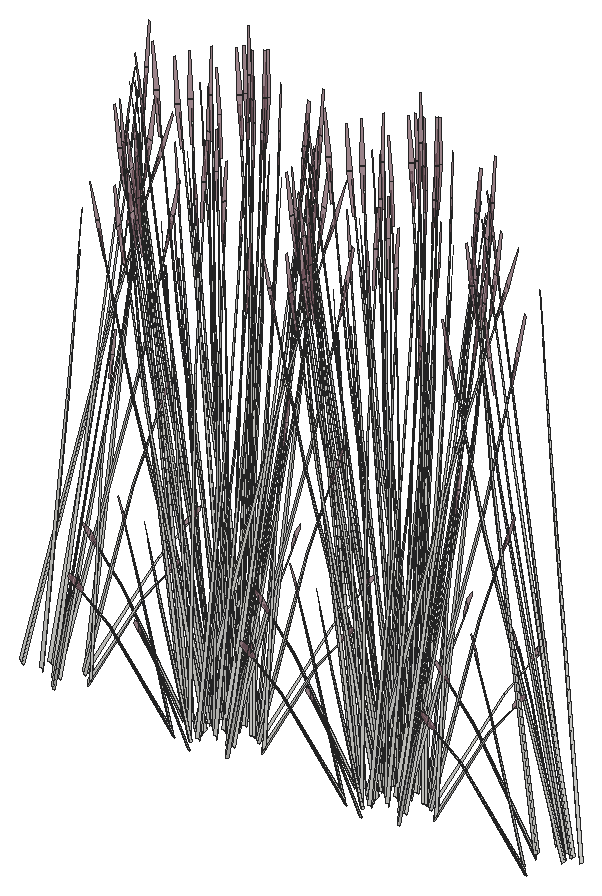
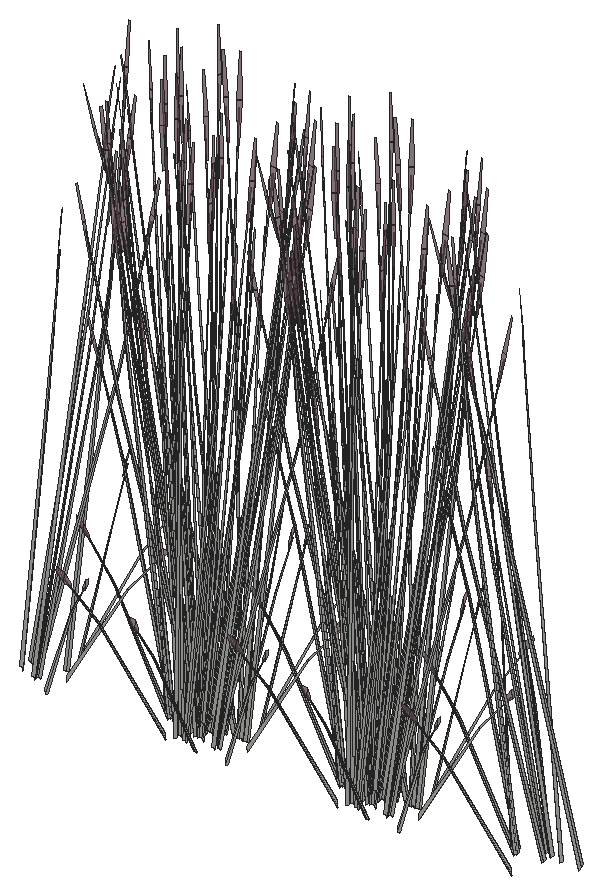
# SketchUp Ruby script. Lengths in inches.
U = 1.inch
M = Sketchup.active_model
def pt(a) = Geom::Point3d.new(a.map { |v| v * U })
def face(e, loops, mat)
  f = e.add_face(loops[0].map { |a| pt(a) })
  loops[1..].each { |l| e.add_face(l.map { |a| pt(a) }).erase! }
  f.material = f.back_material = mat if mat
  f
end
# faces: each face lists its corners as indices into pts; further lists are holes
def faces(e, pts, list, mat = nil) = list.each { |f| face(e, (f[0].is_a?(Array) ? f : [f]).map { |l| l.map { |i| pts[i] } }, mat) }
# xy, xz, yz: faces in a plane at the given z, y or x. An outline is a flat list of corners, or four numbers for a rectangle; further outlines are holes
def ring(l) = l.size == 4 ? [[l[0], l[1]], [l[2], l[1]], [l[2], l[3]], [l[0], l[3]]] : l.each_slice(2).to_a
def flat(e, list, mat, &to3) = list.each { |f| face(e, (f[0].is_a?(Array) ? f : [f]).map { |l| ring(l).map { |u, v| to3.(u, v) } }, mat) }
def xy(e, z, list, mat = nil) = flat(e, list, mat) { |x, y| [x, y, z] }
def xz(e, y, list, mat = nil) = flat(e, list, mat) { |x, z| [x, y, z] }
def yz(e, x, list, mat = nil) = flat(e, list, mat) { |y, z| [x, y, z] }
def lines(e, pts, list) = list.each { |a, b| e.add_line(pt(pts[a]), pt(pts[b])) }
# prism: a flat outline (further loops are holes) pulled along v
def prism(e, loops, v, mat = nil)
  f = face(e, loops, mat); d = Geom::Vector3d.new(v.map { |x| x * U })
  f.pushpull(f.normal.samedirection?(d) ? d.length : -d.length)
end
def box(e, o, s, mat = nil) = prism(e, [[o, [o[0] + s[0], o[1], o[2]], [o[0] + s[0], o[1] + s[1], o[2]], [o[0], o[1] + s[1], o[2]]]], [0, 0, s[2]], mat)
def at(x, y, z, deg = 0) = Geom::Transformation.translation(pt([x, y, z])) * Geom::Transformation.rotation(ORIGIN, Z_AXIS, deg.degrees)
def axes(o, x, y, z) = Geom::Transformation.new([*x, 0, *y, 0, *z, 0, *pt(o).to_a, 1])
def part(name) = M.definitions.add(name)
# library, detail: a bought-in or finely detailed component or shape, given as its bounding box
def library(name, o, s) = part(name).tap { |d| box(d.entities, o, s) }
def detail(e, o, s) = box(e.add_group.entities, o, s)
def put(e, d, t, mat = nil) = e.add_instance(d, t).tap { |i| i.material = mat if mat }
def group(e, t, mat = nil) = e.add_group.tap { |g| g.transformation = t; g.material = mat if mat }.entities
root = M.entities
M.materials.add("LightPink_Translucent").color = [144, 107, 117]
M.materials["LightPink_Translucent"].alpha = 0.75
c1 = part("blade")
p = [[2.15,0.21,22],[0,0.17,0],[0.09,0.45,0],[2.18,0.31,22],[2.29,0.31,22],[0.38,0.45,0],
  [2.48,0.24,33],[2.49,0.24,33],[2.48,0.22,33]]
faces(c1.entities,p,[[0,1,2,3],[4,5,2,3],[6,3,4,7],[8,0,3,6]])
c2 = part("seeds")
p = [[0.3,-0.1,1.38],[-0.01,-0.03,1.59],[-0.01,-0.03,0.03],[0.14,-0.07,-0.07],[0.29,-0.03,3],[0.15,0.01,3.11]]
faces(c2.entities,p,[[0,1,2,3],[1,0,4,5]],"LightPink_Translucent")
c3 = part("blade with seeds")
put(c3.entities,c1,at(0,0,0))
put(c3.entities,c2,axes([2.4,0.25,30.99],[1.5799,-0.05474,1.17369],[-0.12525,1.92788,0.29478],[-0.07173,-0.02425,1.56792]))
put(root,c3,axes([309.91,52.51,257.06],[0.51177,-0.45928,-0.62353],[0.63575,0.41646,-0.16365],[0.20507,-0.11457,1.37633]))
put(root,c3,axes([312.16,52.1,257.03],[0.17848,0.53243,-0.30978],[-0.70886,0.15119,0.30978],[0.1429,0.0614,1.38974]))
put(root,c3,axes([313.49,53.84,257.375],[0.95008,0,0],[0,0.68292,-0.51607],[0,0.15554,1.63711]))
put(root,c3,axes([310.42,52.95,257.67],[0.76714,-0.40567,-0.29095],[0.51013,0.57321,-0.50002],[0.18927,0.05821,1.59708]))
put(root,c3,axes([308.49,52.59,256.59],[-0.74787,0.24464,1.28929],[-0.23804,-0.70192,0.50096],[0.45924,0.01168,1.46642]))
put(root,c3,axes([311.92,51.51,257.375],[0.47504,-0.61229,0],[0.79476,0.34146,-0.51607],[0.18101,0.07777,1.63711]))
put(root,c3,axes([312.72,51.24,256.49],[-0.11372,-0.04814,1.76342],[-0.29211,-0.53779,-0.26939],[0.19706,-0.14594,0.30037]))
put(root,c3,axes([312.36,51.875,257.02],[0.7111,0.30552,-0.49651],[-0.42504,0.54784,0],[0.16196,0.06958,1.57504]))
put(root,c3,axes([312.32,56.22,256.49],[0.05536,-0.08822,1.76342],[0.69692,-0.25981,-0.26939],[0.21129,0.13447,0.30037]))
put(root,c3,axes([311.32,53.05,257.06],[0.79037,0.10018,-0.62353],[-0.16679,0.61794,-0.16365],[0.23587,0.07488,1.37633]))
put(root,c3,axes([314.6875,53.41,257.26],[-0.47106,-0.39072,-0.06488],[0.51591,-0.35801,-0.29416],[0.14618,-0.02521,0.97024]))
put(root,c3,axes([324.24,53.45,256.49],[0.01927,0.0963,1.76342],[-0.38846,0.5029,-0.26939],[-0.27592,-0.02535,0.30037]))
put(root,c3,axes([313.79,53.93,256.98],[-0.48937,0.07333,1.41583],[-0.07789,-0.58369,0.08104],[0.34275,-0.08835,0.80566]))
put(root,c3,axes([314.33,53.55,256.49],[-0.03971,-0.09277,1.76342],[0.27541,-0.54264,-0.26939],[0.27782,-0.00781,0.30037]))
put(root,c3,axes([324.03,56.15,256.49],[0.10192,0.06105,1.76342],[0.17281,0.56562,-0.26939],[-0.22588,0.12062,0.30037]))
put(root,c3,axes([326.78,54.32,257.06],[-0.79037,-0.10018,-0.62353],[0.16679,-0.61794,-0.16365],[-0.23587,-0.07488,1.37633]))
put(root,c3,axes([325.74,55.49,257.02],[-0.7111,-0.30552,-0.49651],[0.42504,-0.54784,0],[-0.16196,-0.06958,1.57504]))
put(root,c3,axes([325.43,50.94,256.49],[-0.0736,0.08049,1.76342],[-0.74378,0.17355,-0.26939],[-0.17968,-0.15788,0.30037]))
put(root,c3,axes([326.17,55.86,257.375],[-0.47504,0.61229,0],[-0.79476,-0.34146,-0.51607],[-0.18101,-0.07777,1.63711]))
put(root,c3,axes([324.97,51.25,257.13],[-0.21918,0.49894,-0.03893],[-0.6746,-0.15348,-0.17649],[-0.10242,-0.08161,0.58215]))
put(root,c3,axes([327.67,54.42,257.67],[-0.76714,0.40567,-0.29095],[-0.51013,-0.57321,-0.50002],[-0.18927,-0.05821,1.59708]))
put(root,c3,axes([324.6,53.53,257.375],[-0.95008,0,0],[0,-0.68292,-0.51607],[0,-0.15554,1.63711]))
put(root,c3,axes([325.9375,55.27,257.03],[-0.17848,-0.53243,-0.30978],[0.70886,-0.15119,0.30978],[-0.1429,-0.0614,1.38974]))
put(root,c3,axes([328.18,54.86,257.06],[-0.51177,0.45928,-0.62353],[-0.63575,-0.41646,-0.16365],[-0.20507,0.11457,1.37633]))
put(root,c3,axes([325.34,53.35,257.33],[-0.70674,0.51372,0.30756],[-0.70717,-0.50832,-0.36492],[-0.02468,-0.14589,1.64885]))
put(root,c3,axes([328.54,54.6,257.46],[-0.74193,-0.49181,-0.25192],[0.6243,-0.55226,0.5513],[-0.19979,0.05753,1.68216]))
put(root,c3,axes([327.1875,54.13,257.21],[-0.45644,-0.51287,-0.44739],[0.69137,-0.36116,0.21531],[-0.14771,-0.06346,1.43643]))
put(root,c3,axes([328.16,54.5,257.21],[-0.82508,0.03772,-0.44739],[-0.07462,-0.62614,0.21531],[-0.14771,0.06346,1.43643]))
put(root,c3,axes([327.25,54.42,257.4375],[0.20138,-0.72405,-0.23429],[0.95485,0.12621,0.51271],[-0.16685,-0.09999,1.5644]))
put(root,c3,axes([329.03,56.11,257.02],[-0.7111,0.30552,-0.49651],[-0.42504,-0.54784,0],[-0.16196,0.06958,1.57504]))
put(root,c3,axes([324.82,53.07,257.02],[0,-0.61104,-0.49651],[0.85008,0,0],[0,-0.13917,1.57504]))
put(root,c3,axes([329.07,55.95,257.19],[-0.46912,-0.61443,-0.05142],[0.79476,-0.34146,0.51607],[-0.19584,0.0585,1.6363]))
put(root,c3,axes([328.86,55.87,257.03],[-0.70886,-0.15119,-0.30978],[0.17848,-0.53243,0.30978],[-0.1429,0.0614,1.38974]))
put(root,c3,axes([327.04,53.77,257.67],[-0.85568,-0.29155,-0.29095],[0.41201,-0.61537,-0.50002],[-0.02689,-0.15109,1.59708]))
put(root,c3,axes([328.74,54.33,257.67],[0.08854,0.69723,-0.29095],[-0.92215,0.04216,-0.50002],[-0.16238,0.09287,1.59708]))
put(root,c3,axes([326.66,53.15,257.1],[-0.31203,-0.62659,-0.69835],[0.89884,-0.22566,-0.18329],[-0.03449,-0.21218,1.54149]))
put(root,c3,axes([325.18,53.08,257.03],[0.53038,-0.38124,-0.30978],[0.53038,0.38124,0.30978],[0,-0.1228,1.38974]))
put(root,c3,axes([327.58,50.62,257.13],[-0.52505,0.35054,-0.03893],[-0.48109,-0.38392,-0.17649],[-0.03387,-0.10878,0.58215]))
put(root,c3,axes([327.9,55.33,257.2],[-0.76598,-0.27433,0],[0.36864,-0.57001,0],[0,0,1.62707]))
put(root,c3,axes([329.67,56.02,257.375],[0.47504,0.61229,0],[-0.79476,0.34146,-0.51607],[-0.18101,0.07777,1.63711]))
put(root,c3,axes([328.71,54.01,257.3],[-0.70674,-0.52593,-0.06131],[0.70717,-0.52625,0],[-0.02468,-0.01837,1.75571]))
put(root,c3,axes([329.1,55.63,257.33],[0.95122,0.19861,0.30756],[-0.23797,0.7099,-0.36492],[-0.15744,0.08885,1.64885]))
put(root,c3,axes([327.71,50.1875,256.49],[-0.12744,0.02202,1.76342],[-0.70477,-0.24781,-0.26939],[0.01183,-0.2067,0.30037]))
put(root,c3,axes([327.13,53.32,257.21],[0.36864,-0.55059,-0.44739],[0.76598,0.26498,0.21531],[0,-0.12692,1.43643]))
put(root,c3,axes([328.08,55.09,257.2],[-0.24791,-0.5268,0],[0.70791,-0.18448,0],[0,0,1.54371]))
put(root,c3,axes([327.17,56.2,256.49],[0.12297,-0.03325,1.76342],[0.73967,0.18301,-0.26939],[0.02163,0.20626,0.30037]))
put(root,c3,axes([329.08,54.05,257.21],[-0.36864,0.55059,-0.44739],[-0.76598,-0.26498,0.21531],[0,0.12692,1.43643]))
put(root,c3,axes([328.47,53.46,257.21],[0,-0.70701,0],[0.95008,0,0],[0,0,1.79456]))
put(root,c3,axes([328.95,53.74,257.29],[0,0.70667,-0.05637],[-0.95008,0,0],[0,0.02221,1.79368]))
put(root,c3,axes([328.49,55.11,257.29],[0.33034,0.70197,-0.06012],[-0.94388,0.24598,0],[0.01154,0.02451,1.72173]))
put(root,c3,axes([326.53,51.35,257.375],[-0.47504,-0.61229,0],[0.79476,-0.34146,-0.51607],[0.18101,-0.07777,1.63711]))
put(root,c3,axes([331.22,54.19,257.2],[-0.94962,-0.00489,-0.04976],[0,-0.68292,0.49943],[-0.02984,0.15546,1.58352]))
put(root,c3,axes([329.1,53.89,257.21],[0.53038,0.39469,0],[-0.53038,0.39469,0],[0,0,1.69266]))
put(root,c3,axes([328.77,55.34,257.2],[0.76598,0.27433,0],[-0.36864,0.57001,0],[0,0,1.74954]))
put(root,c3,axes([331.02,54.29,257.03],[-0.53038,0.38124,-0.30978],[-0.53038,-0.38124,0.30978],[0,0.1228,1.38974]))
put(root,c3,axes([329.51,54.22,257.09],[0.2786,0.55945,-0.69212],[-0.80253,0.20149,-0.18165],[0.03079,0.18945,1.52773]))
put(root,c3,axes([329.12,53.62,257.21],[0.85008,0,0],[0,0.63259,0],[0,0,1.78407]))
put(root,c3,axes([327.47,53.04,257.67],[-0.08854,-0.69723,-0.29095],[0.92215,-0.04216,-0.50002],[0.16238,-0.09287,1.59708]))
put(root,c3,axes([329.17,53.6,257.67],[0.85568,0.29155,-0.29095],[-0.41201,0.61537,-0.50002],[0.02689,0.15109,1.59708]))
put(root,c3,axes([327.35,51.5,257.03],[0.70886,0.15119,-0.30978],[-0.17848,0.53243,0.30978],[0.1429,-0.0614,1.38974]))
put(root,c3,axes([331.39,54.3,257.02],[0,0.61104,-0.49651],[-0.85008,0,0],[0,0.13917,1.57504]))
put(root,c3,axes([327.18,51.26,257.02],[0.7111,-0.30552,-0.49651],[0.42504,0.54784,0],[0.16196,-0.06958,1.57504]))
put(root,c3,axes([329,55.02,257.18],[0.79769,-0.20732,-0.19198],[0.2803,0.59721,0.00008],[0.08805,-0.02292,1.73897]))
put(root,c3,axes([329.02,53.24,257.21],[0.45644,0.51287,-0.44739],[-0.69137,0.36116,0.21531],[0.14771,0.06346,1.43643]))
put(root,c3,axes([328.02,52.51,257.06],[0.51177,-0.45928,-0.62353],[0.63575,0.41646,-0.16365],[0.20507,-0.11457,1.37633]))
put(root,c3,axes([330.27,52.1,257.03],[0.17848,0.53243,-0.30978],[-0.70886,0.15119,0.30978],[0.1429,0.0614,1.38974]))
put(root,c3,axes([331.6,53.84,257.375],[0.95008,0,0],[0,0.68292,-0.51607],[0,0.15554,1.63711]))
put(root,c3,axes([328.53,52.95,257.67],[0.76714,-0.40567,-0.29095],[0.51013,0.57321,-0.50002],[0.18927,0.05821,1.59708]))
put(root,c3,axes([326.59,52.59,256.59],[-0.74787,0.24464,1.28929],[-0.23804,-0.70192,0.50096],[0.45924,0.01168,1.46642]))
put(root,c3,axes([330.03,51.51,257.375],[0.47504,-0.61229,0],[0.79476,0.34146,-0.51607],[0.18101,0.07777,1.63711]))
put(root,c3,axes([330.83,51.24,256.49],[-0.11372,-0.04814,1.76342],[-0.29211,-0.53779,-0.26939],[0.19706,-0.14594,0.30037]))
put(root,c3,axes([330.47,51.875,257.02],[0.7111,0.30552,-0.49651],[-0.42504,0.54784,0],[0.16196,0.06958,1.57504]))
put(root,c3,axes([330.43,56.22,256.49],[0.05536,-0.08822,1.76342],[0.69692,-0.25981,-0.26939],[0.21129,0.13447,0.30037]))
put(root,c3,axes([329.43,53.05,257.06],[0.79037,0.10018,-0.62353],[-0.16679,0.61794,-0.16365],[0.23587,0.07488,1.37633]))
put(root,c3,axes([332.79,53.41,257.26],[-0.47106,-0.39072,-0.06488],[0.51591,-0.35801,-0.29416],[0.14618,-0.02521,0.97024]))
put(root,c3,axes([342.14,53.45,256.49],[0.01927,0.0963,1.76342],[-0.38846,0.5029,-0.26939],[-0.27592,-0.02535,0.30037]))
put(root,c3,axes([331.9,53.93,256.98],[-0.48937,0.07333,1.41583],[-0.07789,-0.58369,0.08104],[0.34275,-0.08835,0.80566]))
put(root,c3,axes([332.4375,53.55,256.49],[-0.03971,-0.09277,1.76342],[0.27541,-0.54264,-0.26939],[0.27782,-0.00781,0.30037]))
put(root,c3,axes([341.94,56.15,256.49],[0.10192,0.06105,1.76342],[0.17281,0.56562,-0.26939],[-0.22588,0.12062,0.30037]))
put(root,c3,axes([344.68,54.32,257.06],[-0.79037,-0.10018,-0.62353],[0.16679,-0.61794,-0.16365],[-0.23587,-0.07488,1.37633]))
put(root,c3,axes([343.65,55.49,257.02],[-0.7111,-0.30552,-0.49651],[0.42504,-0.54784,0],[-0.16196,-0.06958,1.57504]))
put(root,c3,axes([343.34,50.94,256.49],[-0.0736,0.08049,1.76342],[-0.74378,0.17355,-0.26939],[-0.17968,-0.15788,0.30037]))
put(root,c3,axes([344.08,55.86,257.375],[-0.47504,0.61229,0],[-0.79476,-0.34146,-0.51607],[-0.18101,-0.07777,1.63711]))
put(root,c3,axes([342.875,51.25,257.13],[-0.21918,0.49894,-0.03893],[-0.6746,-0.15348,-0.17649],[-0.10242,-0.08161,0.58215]))
put(root,c3,axes([345.58,54.42,257.67],[-0.76714,0.40567,-0.29095],[-0.51013,-0.57321,-0.50002],[-0.18927,-0.05821,1.59708]))
put(root,c3,axes([342.51,53.53,257.375],[-0.95008,0,0],[0,-0.68292,-0.51607],[0,-0.15554,1.63711]))
put(root,c3,axes([343.85,55.27,257.03],[-0.17848,-0.53243,-0.30978],[0.70886,-0.15119,0.30978],[-0.1429,-0.0614,1.38974]))
put(root,c3,axes([346.09,54.86,257.06],[-0.51177,0.45928,-0.62353],[-0.63575,-0.41646,-0.16365],[-0.20507,0.11457,1.37633]))
put(root,c3,axes([343.25,53.35,257.33],[-0.70674,0.51372,0.30756],[-0.70717,-0.50832,-0.36492],[-0.02468,-0.14589,1.64885]))
put(root,c3,axes([346.44,54.6,257.46],[-0.74193,-0.49181,-0.25192],[0.6243,-0.55226,0.5513],[-0.19979,0.05753,1.68216]))
put(root,c3,axes([345.09,54.13,257.21],[-0.45644,-0.51287,-0.44739],[0.69137,-0.36116,0.21531],[-0.14771,-0.06346,1.43643]))
put(root,c3,axes([346.07,54.5,257.21],[-0.82508,0.03772,-0.44739],[-0.07462,-0.62614,0.21531],[-0.14771,0.06346,1.43643]))
put(root,c3,axes([345.16,54.42,257.4375],[0.20138,-0.72405,-0.23429],[0.95485,0.12621,0.51271],[-0.16685,-0.09999,1.5644]))
put(root,c3,axes([346.93,56.11,257.02],[-0.7111,0.30552,-0.49651],[-0.42504,-0.54784,0],[-0.16196,0.06958,1.57504]))
put(root,c3,axes([342.72,53.07,257.02],[0,-0.61104,-0.49651],[0.85008,0,0],[0,-0.13917,1.57504]))
put(root,c3,axes([346.98,55.95,257.19],[-0.46912,-0.61443,-0.05142],[0.79476,-0.34146,0.51607],[-0.19584,0.0585,1.6363]))
put(root,c3,axes([346.77,55.87,257.03],[-0.70886,-0.15119,-0.30978],[0.17848,-0.53243,0.30978],[-0.1429,0.0614,1.38974]))
put(root,c3,axes([344.95,53.77,257.67],[-0.85568,-0.29155,-0.29095],[0.41201,-0.61537,-0.50002],[-0.02689,-0.15109,1.59708]))
put(root,c3,axes([346.65,54.33,257.67],[0.08854,0.69723,-0.29095],[-0.92215,0.04216,-0.50002],[-0.16238,0.09287,1.59708]))
put(root,c3,axes([344.5625,53.15,257.1],[-0.31203,-0.62659,-0.69835],[0.89884,-0.22566,-0.18329],[-0.03449,-0.21218,1.54149]))
put(root,c3,axes([343.09,53.08,257.03],[0.53038,-0.38124,-0.30978],[0.53038,0.38124,0.30978],[0,-0.1228,1.38974]))
put(root,c3,axes([345.48,50.62,257.13],[-0.52505,0.35054,-0.03893],[-0.48109,-0.38392,-0.17649],[-0.03387,-0.10878,0.58215]))
put(root,c3,axes([345.81,55.33,257.2],[-0.76598,-0.27433,0],[0.36864,-0.57001,0],[0,0,1.62707]))
put(root,c3,axes([347.58,56.02,257.375],[0.47504,0.61229,0],[-0.79476,0.34146,-0.51607],[-0.18101,0.07777,1.63711]))
put(root,c3,axes([346.61,54.01,257.3],[-0.70674,-0.52593,-0.06131],[0.70717,-0.52625,0],[-0.02468,-0.01837,1.75571]))
put(root,c3,axes([347,55.63,257.33],[0.95122,0.19861,0.30756],[-0.23797,0.7099,-0.36492],[-0.15744,0.08885,1.64885]))
put(root,c3,axes([345.61,50.1875,256.49],[-0.12744,0.02202,1.76342],[-0.70477,-0.24781,-0.26939],[0.01183,-0.2067,0.30037]))
put(root,c3,axes([345.04,53.32,257.21],[0.36864,-0.55059,-0.44739],[0.76598,0.26498,0.21531],[0,-0.12692,1.43643]))
put(root,c3,axes([345.98,55.09,257.2],[-0.24791,-0.5268,0],[0.70791,-0.18448,0],[0,0,1.54371]))
put(root,c3,axes([345.08,56.2,256.49],[0.12297,-0.03325,1.76342],[0.73967,0.18301,-0.26939],[0.02163,0.20626,0.30037]))
put(root,c3,axes([346.98,54.05,257.21],[-0.36864,0.55059,-0.44739],[-0.76598,-0.26498,0.21531],[0,0.12692,1.43643]))
put(root,c3,axes([346.375,53.46,257.21],[0,-0.70701,0],[0.95008,0,0],[0,0,1.79456]))
put(root,c3,axes([346.85,53.74,257.29],[0,0.70667,-0.05637],[-0.95008,0,0],[0,0.02221,1.79368]))
put(root,c3,axes([346.4,55.11,257.29],[0.33034,0.70197,-0.06012],[-0.94388,0.24598,0],[0.01154,0.02451,1.72173]))
put(root,c3,axes([344.44,51.35,257.375],[-0.47504,-0.61229,0],[0.79476,-0.34146,-0.51607],[0.18101,-0.07777,1.63711]))
put(root,c3,axes([349.13,54.19,257.2],[-0.94962,-0.00489,-0.04976],[0,-0.68292,0.49943],[-0.02984,0.15546,1.58352]))
put(root,c3,axes([347,53.89,257.21],[0.53038,0.39469,0],[-0.53038,0.39469,0],[0,0,1.69266]))
put(root,c3,axes([346.68,55.34,257.2],[0.76598,0.27433,0],[-0.36864,0.57001,0],[0,0,1.74954]))
put(root,c3,axes([348.93,54.29,257.03],[-0.53038,0.38124,-0.30978],[-0.53038,-0.38124,0.30978],[0,0.1228,1.38974]))
put(root,c3,axes([347.42,54.22,257.09],[0.2786,0.55945,-0.69212],[-0.80253,0.20149,-0.18165],[0.03079,0.18945,1.52773]))
put(root,c3,axes([347.02,53.62,257.21],[0.85008,0,0],[0,0.63259,0],[0,0,1.78407]))
put(root,c3,axes([345.375,53.04,257.67],[-0.08854,-0.69723,-0.29095],[0.92215,-0.04216,-0.50002],[0.16238,-0.09287,1.59708]))
put(root,c3,axes([347.07,53.6,257.67],[0.85568,0.29155,-0.29095],[-0.41201,0.61537,-0.50002],[0.02689,0.15109,1.59708]))
put(root,c3,axes([345.25,51.5,257.03],[0.70886,0.15119,-0.30978],[-0.17848,0.53243,0.30978],[0.1429,-0.0614,1.38974]))
put(root,c3,axes([349.3,54.3,257.02],[0,0.61104,-0.49651],[-0.85008,0,0],[0,0.13917,1.57504]))
put(root,c3,axes([345.09,51.26,257.02],[0.7111,-0.30552,-0.49651],[0.42504,0.54784,0],[0.16196,-0.06958,1.57504]))
put(root,c3,axes([346.91,55.02,257.18],[0.79769,-0.20732,-0.19198],[0.2803,0.59721,0.00008],[0.08805,-0.02292,1.73897]))
put(root,c3,axes([346.92,53.24,257.21],[0.45644,0.51287,-0.44739],[-0.69137,0.36116,0.21531],[0.14771,0.06346,1.43643]))
put(root,c3,axes([345.93,52.51,257.06],[0.51177,-0.45928,-0.62353],[0.63575,0.41646,-0.16365],[0.20507,-0.11457,1.37633]))
put(root,c3,axes([348.17,52.1,257.03],[0.17848,0.53243,-0.30978],[-0.70886,0.15119,0.30978],[0.1429,0.0614,1.38974]))
put(root,c3,axes([349.51,53.84,257.375],[0.95008,0,0],[0,0.68292,-0.51607],[0,0.15554,1.63711]))
put(root,c3,axes([346.4375,52.95,257.67],[0.76714,-0.40567,-0.29095],[0.51013,0.57321,-0.50002],[0.18927,0.05821,1.59708]))
put(root,c3,axes([344.5,52.59,256.59],[-0.74787,0.24464,1.28929],[-0.23804,-0.70192,0.50096],[0.45924,0.01168,1.46642]))
put(root,c3,axes([347.9375,51.51,257.375],[0.47504,-0.61229,0],[0.79476,0.34146,-0.51607],[0.18101,0.07777,1.63711]))
put(root,c3,axes([348.73,51.24,256.49],[-0.11372,-0.04814,1.76342],[-0.29211,-0.53779,-0.26939],[0.19706,-0.14594,0.30037]))
put(root,c3,axes([348.37,51.875,257.02],[0.7111,0.30552,-0.49651],[-0.42504,0.54784,0],[0.16196,0.06958,1.57504]))
put(root,c3,axes([348.34,56.22,256.49],[0.05536,-0.08822,1.76342],[0.69692,-0.25981,-0.26939],[0.21129,0.13447,0.30037]))
put(root,c3,axes([347.33,53.05,257.06],[0.79037,0.10018,-0.62353],[-0.16679,0.61794,-0.16365],[0.23587,0.07488,1.37633]))
put(root,c3,axes([350.7,53.41,257.26],[-0.47106,-0.39072,-0.06488],[0.51591,-0.35801,-0.29416],[0.14618,-0.02521,0.97024]))
put(root,c3,axes([349.81,53.93,256.98],[-0.48937,0.07333,1.41583],[-0.07789,-0.58369,0.08104],[0.34275,-0.08835,0.80566]))
put(root,c3,axes([350.34,53.55,256.49],[-0.03971,-0.09277,1.76342],[0.27541,-0.54264,-0.26939],[0.27782,-0.00781,0.30037]))
put(root,c3,axes([360.93,53.45,256.49],[0.01927,0.0963,1.76342],[-0.38846,0.5029,-0.26939],[-0.27592,-0.02535,0.30037]))
put(root,c3,axes([360.72,56.15,256.49],[0.10192,0.06105,1.76342],[0.17281,0.56562,-0.26939],[-0.22588,0.12062,0.30037]))
put(root,c3,axes([363.47,54.32,257.06],[-0.79037,-0.10018,-0.62353],[0.16679,-0.61794,-0.16365],[-0.23587,-0.07488,1.37633]))
put(root,c3,axes([362.43,55.49,257.02],[-0.7111,-0.30552,-0.49651],[0.42504,-0.54784,0],[-0.16196,-0.06958,1.57504]))
put(root,c3,axes([362.12,50.94,256.49],[-0.0736,0.08049,1.76342],[-0.74378,0.17355,-0.26939],[-0.17968,-0.15788,0.30037]))
put(root,c3,axes([362.86,55.86,257.375],[-0.47504,0.61229,0],[-0.79476,-0.34146,-0.51607],[-0.18101,-0.07777,1.63711]))
put(root,c3,axes([361.66,51.25,257.13],[-0.21918,0.49894,-0.03893],[-0.6746,-0.15348,-0.17649],[-0.10242,-0.08161,0.58215]))
put(root,c3,axes([364.36,54.42,257.67],[-0.76714,0.40567,-0.29095],[-0.51013,-0.57321,-0.50002],[-0.18927,-0.05821,1.59708]))
put(root,c3,axes([361.29,53.53,257.375],[-0.95008,0,0],[0,-0.68292,-0.51607],[0,-0.15554,1.63711]))
put(root,c3,axes([362.63,55.27,257.03],[-0.17848,-0.53243,-0.30978],[0.70886,-0.15119,0.30978],[-0.1429,-0.0614,1.38974]))
put(root,c3,axes([364.875,54.86,257.06],[-0.51177,0.45928,-0.62353],[-0.63575,-0.41646,-0.16365],[-0.20507,0.11457,1.37633]))
